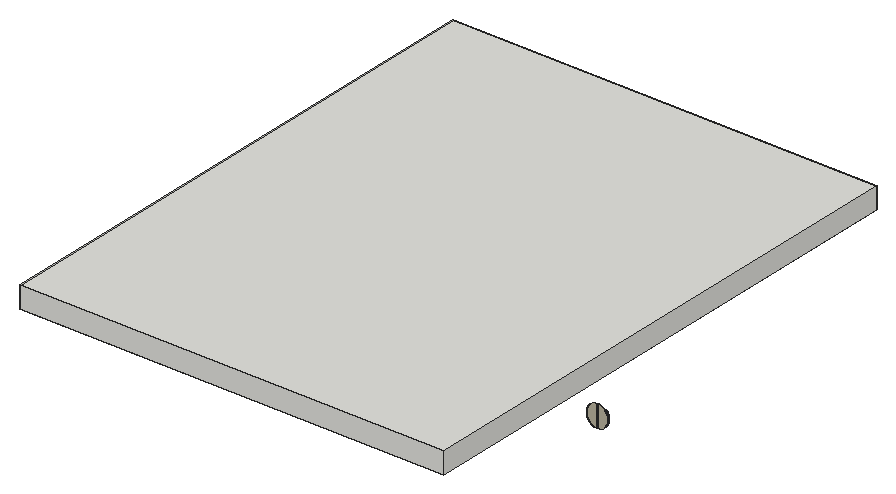
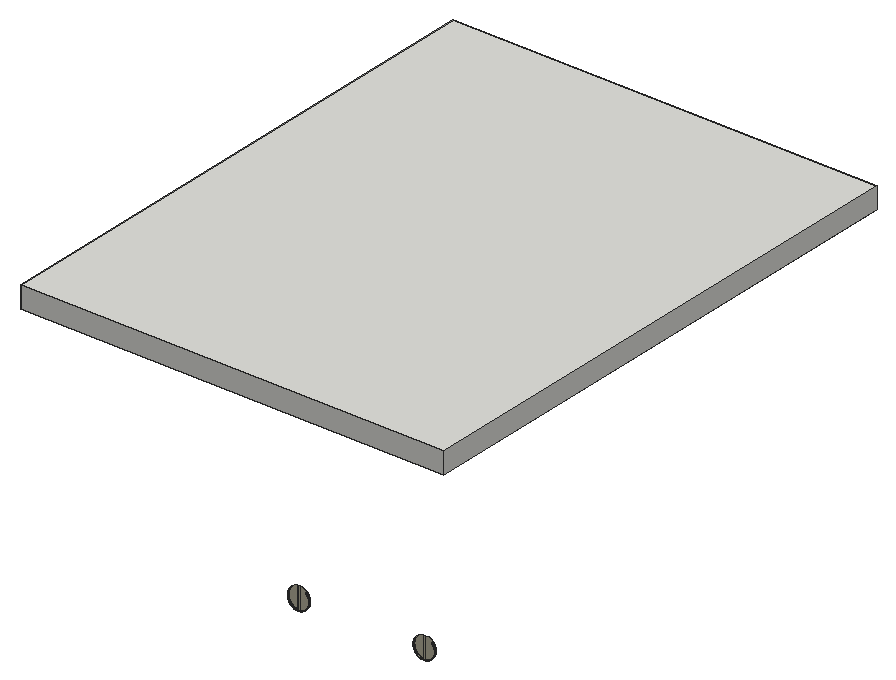
# SketchUp Ruby script. Lengths in millimetres.
U = 1.mm
M = Sketchup.active_model
def pt(a) = Geom::Point3d.new(a.map { |v| v * U })
def face(e, loops, mat)
  f = e.add_face(loops[0].map { |a| pt(a) })
  loops[1..].each { |l| e.add_face(l.map { |a| pt(a) }).erase! }
  f.material = f.back_material = mat if mat
  f
end
# faces: each face lists its corners as indices into pts; further lists are holes
def faces(e, pts, list, mat = nil) = list.each { |f| face(e, (f[0].is_a?(Array) ? f : [f]).map { |l| l.map { |i| pts[i] } }, mat) }
# xy, xz, yz: faces in a plane at the given z, y or x. An outline is a flat list of corners, or four numbers for a rectangle; further outlines are holes
def ring(l) = l.size == 4 ? [[l[0], l[1]], [l[2], l[1]], [l[2], l[3]], [l[0], l[3]]] : l.each_slice(2).to_a
def flat(e, list, mat, &to3) = list.each { |f| face(e, (f[0].is_a?(Array) ? f : [f]).map { |l| ring(l).map { |u, v| to3.(u, v) } }, mat) }
def xy(e, z, list, mat = nil) = flat(e, list, mat) { |x, y| [x, y, z] }
def xz(e, y, list, mat = nil) = flat(e, list, mat) { |x, z| [x, y, z] }
def yz(e, x, list, mat = nil) = flat(e, list, mat) { |y, z| [x, y, z] }
def lines(e, pts, list) = list.each { |a, b| e.add_line(pt(pts[a]), pt(pts[b])) }
# prism: a flat outline (further loops are holes) pulled along v
def prism(e, loops, v, mat = nil)
  f = face(e, loops, mat); d = Geom::Vector3d.new(v.map { |x| x * U })
  f.pushpull(f.normal.samedirection?(d) ? d.length : -d.length)
end
def box(e, o, s, mat = nil) = prism(e, [[o, [o[0] + s[0], o[1], o[2]], [o[0] + s[0], o[1] + s[1], o[2]], [o[0], o[1] + s[1], o[2]]]], [0, 0, s[2]], mat)
def at(x, y, z, deg = 0) = Geom::Transformation.translation(pt([x, y, z])) * Geom::Transformation.rotation(ORIGIN, Z_AXIS, deg.degrees)
def axes(o, x, y, z) = Geom::Transformation.new([*x, 0, *y, 0, *z, 0, *pt(o).to_a, 1])
def part(name) = M.definitions.add(name)
# library, detail: a bought-in or finely detailed component or shape, given as its bounding box
def library(name, o, s) = part(name).tap { |d| box(d.entities, o, s) }
def detail(e, o, s) = box(e.add_group.entities, o, s)
def put(e, d, t, mat = nil) = e.add_instance(d, t).tap { |i| i.material = mat if mat }
def group(e, t, mat = nil) = e.add_group.tap { |g| g.transformation = t; g.material = mat if mat }.entities
root = M.entities
M.materials.add("Uniboard-L19-Putty-4K").color = [187, 181, 160]
M.materials.add("[Color M09]").color = [0, 0, 0]
c1 = part("Group\#7")
detail(c1.entities,[0,0,0],[98.4,98.4,20])
xy(root,1219.2,[[604.4,3403.6,618.1,3413.6],[621.1,3403.6,634.7,3413.6],[1510.3,3403.6,1524,3413.6],[1527,3403.6,1540.7,3413.6]],"Uniboard-L19-Putty-4K")
xy(root,2871.6,[[1998,3403.6,2410.4,3412.6],[2449.4,3403.6,2861.9,3412.6]],"[Color M09]")
xz(root,3403.6,[[604.4,1219.2,618.1,1219.2,618.1,1371.6,604.4,1371.6,602.6,1371.2,600.2,1370.7,595.6,1369.3,593.2,1368.5,591,1367.6,588.7,1366.7,586.5,1365.7,582.1,1363.5,580,1362.3,577.9,1361,575.9,1359.7,573.9,1358.3,571.9,1356.8,570,1355.3,568.2,1353.7,564.6,1350.3,562.9,1348.6,561.3,1346.8,559.7,1344.9,556.7,1341.1,555.3,1339.1,554,1337,552.7,1335,551.5,1332.8,550.3,1330.7,548.3,1326.3,547.3,1324,545.7,1319.4,545,1317.1,544.3,1314.7,543.7,1312.3,543.2,1310,542.8,1307.6,542.5,1305.1,542.2,1302.7,542,1300.3,541.9,1297.8,541.9,1293,542,1290.5,542.2,1288.1,542.5,1285.7,542.8,1283.2,543.2,1280.8,543.7,1278.5,544.3,1276.1,545,1273.7,545.7,1271.4,547.3,1266.8,548.3,1264.5,550.3,1260.1,551.5,1258,552.7,1255.8,554,1253.8,555.3,1251.7,556.7,1249.7,559.7,1245.9,561.3,1244,562.9,1242.2,564.6,1240.5,568.2,1237.1,570,1235.5,571.9,1234,573.9,1232.5,575.9,1231.1,577.9,1229.8,580,1228.5,582.1,1227.3,586.5,1225.1,588.7,1224.1,591,1223.2,593.2,1222.3,595.6,1221.5,600.2,1220.1,602.6,1219.6],[621.1,1219.2,634.7,1219.2,636.5,1219.6,638.9,1220.1,641.2,1220.8,643.6,1221.5,645.9,1222.3,648.2,1223.2,650.4,1224.1,652.6,1225.1,657,1227.3,659.1,1228.5,661.2,1229.8,663.2,1231.1,665.2,1232.5,667.2,1234,669.1,1235.5,671,1237.1,672.8,1238.8,676.2,1242.2,677.9,1244,679.4,1245.9,681,1247.8,682.4,1249.7,683.8,1251.7,685.2,1253.8,686.4,1255.8,687.7,1258,688.8,1260.1,689.9,1262.3,690.9,1264.5,692.7,1269.1,693.5,1271.4,694.2,1273.7,695.4,1278.5,695.9,1280.8,696.3,1283.2,696.7,1285.7,697.1,1290.5,697.2,1293,697.3,1295.4,697.2,1297.8,697.1,1300.3,696.7,1305.1,696.3,1307.6,695.9,1310,695.4,1312.3,694.2,1317.1,693.5,1319.4,692.7,1321.7,690.9,1326.3,689.9,1328.5,688.8,1330.7,687.7,1332.8,686.4,1335,685.2,1337,683.8,1339.1,682.4,1341.1,681,1343,679.4,1344.9,677.9,1346.8,676.2,1348.6,672.8,1352,671,1353.7,669.1,1355.3,667.2,1356.8,665.2,1358.3,663.2,1359.7,661.2,1361,659.1,1362.3,657,1363.5,652.6,1365.7,650.4,1366.7,648.2,1367.6,645.9,1368.5,643.6,1369.3,641.2,1370,638.9,1370.7,636.5,1371.2,634.7,1371.6,621.1,1371.6],[1510.3,1219.2,1524,1219.2,1524,1371.6,1510.3,1371.6,1508.6,1371.2,1506.2,1370.7,1503.8,1370,1501.5,1369.3,1499.2,1368.5,1494.6,1366.7,1492.4,1365.7,1490.2,1364.6,1488.1,1363.5,1485.9,1362.3,1483.9,1361,1481.8,1359.7,1479.8,1358.3,1476,1355.3,1474.1,1353.7,1472.3,1352,1468.9,1348.6,1467.2,1346.8,1465.6,1344.9,1462.6,1341.1,1461.2,1339.1,1459.9,1337,1458.6,1335,1457.4,1332.8,1456.3,1330.7,1455.2,1328.5,1454.2,1326.3,1452.4,1321.7,1451.6,1319.4,1450.9,1317.1,1450.2,1314.7,1449.7,1312.3,1449.2,1310,1448.8,1307.6,1448.4,1305.1,1448.1,1302.7,1448,1300.3,1447.8,1297.8,1447.8,1293,1448,1290.5,1448.1,1288.1,1448.4,1285.7,1448.8,1283.2,1449.2,1280.8,1449.7,1278.5,1450.2,1276.1,1450.9,1273.7,1451.6,1271.4,1452.4,1269.1,1454.2,1264.5,1455.2,1262.3,1456.3,1260.1,1457.4,1258,1458.6,1255.8,1459.9,1253.8,1461.2,1251.7,1462.6,1249.7,1465.6,1245.9,1467.2,1244,1468.9,1242.2,1472.3,1238.8,1474.1,1237.1,1476,1235.5,1479.8,1232.5,1481.8,1231.1,1483.9,1229.8,1485.9,1228.5,1488.1,1227.3,1490.2,1226.2,1492.4,1225.1,1494.6,1224.1,1499.2,1222.3,1501.5,1221.5,1503.8,1220.8,1506.2,1220.1,1508.6,1219.6],[1527,1219.2,1540.7,1219.2,1542.4,1219.6,1544.8,1220.1,1547.2,1220.8,1549.5,1221.5,1551.8,1222.3,1556.4,1224.1,1558.6,1225.1,1560.8,1226.2,1562.9,1227.3,1565.1,1228.5,1567.1,1229.8,1569.2,1231.1,1571.2,1232.5,1575,1235.5,1576.9,1237.1,1578.7,1238.8,1582.1,1242.2,1583.8,1244,1585.4,1245.9,1588.4,1249.7,1589.8,1251.7,1591.1,1253.8,1592.4,1255.8,1593.6,1258,1594.7,1260.1,1595.8,1262.3,1596.8,1264.5,1598.6,1269.1,1599.4,1271.4,1600.1,1273.7,1600.8,1276.1,1601.3,1278.5,1601.8,1280.8,1602.2,1283.2,1602.6,1285.7,1602.9,1288.1,1603,1290.5,1603.2,1293,1603.2,1297.8,1603,1300.3,1602.9,1302.7,1602.6,1305.1,1602.2,1307.6,1601.8,1310,1601.3,1312.3,1600.8,1314.7,1600.1,1317.1,1599.4,1319.4,1598.6,1321.7,1596.8,1326.3,1595.8,1328.5,1594.7,1330.7,1593.6,1332.8,1592.4,1335,1591.1,1337,1589.8,1339.1,1588.4,1341.1,1585.4,1344.9,1583.8,1346.8,1582.1,1348.6,1578.7,1352,1576.9,1353.7,1575,1355.3,1571.2,1358.3,1569.2,1359.7,1567.1,1361,1565.1,1362.3,1562.9,1363.5,1560.8,1364.6,1558.6,1365.7,1556.4,1366.7,1551.8,1368.5,1549.5,1369.3,1547.2,1370,1544.8,1370.7,1542.4,1371.2,1540.7,1371.6,1527,1371.6]],"Uniboard-L19-Putty-4K")
yz(root,541.9,[[3403.6,1293,3413.6,1295.4],[3403.6,1295.4,3413.6,1297.8]],"Uniboard-L19-Putty-4K")
yz(root,618.1,[[3403.6,1219.2,3413.6,1371.6]],"Uniboard-L19-Putty-4K")
yz(root,621.1,[[3403.6,1219.2,3413.6,1371.6]],"Uniboard-L19-Putty-4K")
yz(root,1447.8,[[3403.6,1293,3413.6,1295.4],[3403.6,1295.4,3413.6,1297.8]],"Uniboard-L19-Putty-4K")
yz(root,1524,[[3403.6,1219.2,3413.6,1371.6]],"Uniboard-L19-Putty-4K")
yz(root,1527,[[3403.6,1219.2,3413.6,1371.6]],"Uniboard-L19-Putty-4K")
yz(root,1603.2,[[3403.6,1293,3413.6,1295.4],[3403.6,1295.4,3413.6,1297.8]])
p = [[602.6,3413.6,1219.6],[604.4,3413.6,1219.2],[604.4,3403.6,1219.2],[602.6,3403.6,1219.6],[634.7,3413.6,1219.2],[636.5,3413.6,1219.6],
  [636.5,3403.6,1219.6],[634.7,3403.6,1219.2],[1508.6,3413.6,1219.6],[1510.3,3413.6,1219.2],[1510.3,3403.6,1219.2],[1508.6,3403.6,1219.6],
  [1540.7,3413.6,1219.2],[1542.4,3413.6,1219.6],[1542.4,3403.6,1219.6],[1540.7,3403.6,1219.2],[600.2,3413.6,1220.1],[600.2,3403.6,1220.1],
  [638.9,3413.6,1220.1],[638.9,3403.6,1220.1],[1506.2,3413.6,1220.1],[1506.2,3403.6,1220.1],[1544.8,3413.6,1220.1],[1544.8,3403.6,1220.1],
  [597.9,3413.6,1220.8],[597.9,3403.6,1220.8],[641.2,3413.6,1220.8],[641.2,3403.6,1220.8],[1503.8,3413.6,1220.8],[1503.8,3403.6,1220.8],
  [1547.2,3413.6,1220.8],[1547.2,3403.6,1220.8],[595.6,3413.6,1221.5],[595.6,3403.6,1221.5],[643.6,3413.6,1221.5],[643.6,3403.6,1221.5],
  [1501.5,3413.6,1221.5],[1501.5,3403.6,1221.5],[1549.5,3413.6,1221.5],[1549.5,3403.6,1221.5],[593.2,3413.6,1222.3],[593.2,3403.6,1222.3],
  [645.9,3413.6,1222.3],[645.9,3403.6,1222.3],[1499.2,3413.6,1222.3],[1499.2,3403.6,1222.3],[1551.8,3413.6,1222.3],[1551.8,3403.6,1222.3],
  [591,3413.6,1223.2],[591,3403.6,1223.2],[648.2,3413.6,1223.2],[648.2,3403.6,1223.2],[1496.9,3413.6,1223.2],[1496.9,3403.6,1223.2],
  [1554.1,3413.6,1223.2],[1554.1,3403.6,1223.2],[588.7,3413.6,1224.1],[588.7,3403.6,1224.1],[650.4,3413.6,1224.1],[650.4,3403.6,1224.1],
  [1494.6,3413.6,1224.1],[1494.6,3403.6,1224.1],[1556.4,3413.6,1224.1],[1556.4,3403.6,1224.1],[586.5,3413.6,1225.1],[586.5,3403.6,1225.1],
  [652.6,3413.6,1225.1],[652.6,3403.6,1225.1],[1492.4,3413.6,1225.1],[1492.4,3403.6,1225.1],[1558.6,3413.6,1225.1],[1558.6,3403.6,1225.1],
  [584.3,3413.6,1226.2],[584.3,3403.6,1226.2],[654.8,3413.6,1226.2],[654.8,3403.6,1226.2],[1490.2,3413.6,1226.2],[1490.2,3403.6,1226.2],
  [1560.8,3413.6,1226.2],[1560.8,3403.6,1226.2],[582.1,3413.6,1227.3],[582.1,3403.6,1227.3],[657,3413.6,1227.3],[657,3403.6,1227.3],
  [1488.1,3413.6,1227.3],[1488.1,3403.6,1227.3],[1562.9,3413.6,1227.3],[1562.9,3403.6,1227.3],[580,3413.6,1228.5],[580,3403.6,1228.5],
  [659.1,3413.6,1228.5],[659.1,3403.6,1228.5],[1485.9,3413.6,1228.5],[1485.9,3403.6,1228.5],[1565.1,3413.6,1228.5],[1565.1,3403.6,1228.5],
  [577.9,3413.6,1229.8],[577.9,3403.6,1229.8],[661.2,3413.6,1229.8],[661.2,3403.6,1229.8],[1483.9,3413.6,1229.8],[1483.9,3403.6,1229.8],
  [1567.1,3413.6,1229.8],[1567.1,3403.6,1229.8],[575.9,3413.6,1231.1],[575.9,3403.6,1231.1],[663.2,3413.6,1231.1],[663.2,3403.6,1231.1],
  [1481.8,3413.6,1231.1],[1481.8,3403.6,1231.1],[1569.2,3413.6,1231.1],[1569.2,3403.6,1231.1],[573.9,3413.6,1232.5],[573.9,3403.6,1232.5],
  [665.2,3413.6,1232.5],[665.2,3403.6,1232.5],[1479.8,3413.6,1232.5],[1479.8,3403.6,1232.5],[1571.2,3413.6,1232.5],[1571.2,3403.6,1232.5],
  [571.9,3413.6,1234],[571.9,3403.6,1234],[667.2,3413.6,1234],[667.2,3403.6,1234],[1477.9,3413.6,1234],[1477.9,3403.6,1234],
  [1573.1,3413.6,1234],[1573.1,3403.6,1234],[570,3413.6,1235.5],[570,3403.6,1235.5],[669.1,3413.6,1235.5],[669.1,3403.6,1235.5],
  [1476,3413.6,1235.5],[1476,3403.6,1235.5],[1575,3413.6,1235.5],[1575,3403.6,1235.5],[568.2,3413.6,1237.1],[568.2,3403.6,1237.1],
  [671,3413.6,1237.1],[671,3403.6,1237.1],[1474.1,3413.6,1237.1],[1474.1,3403.6,1237.1],[1576.9,3413.6,1237.1],[1576.9,3403.6,1237.1],
  [566.4,3413.6,1238.8],[566.4,3403.6,1238.8],[672.8,3413.6,1238.8],[672.8,3403.6,1238.8],[1472.3,3413.6,1238.8],[1472.3,3403.6,1238.8],
  [1578.7,3413.6,1238.8],[1578.7,3403.6,1238.8],[564.6,3413.6,1240.5],[564.6,3403.6,1240.5],[674.5,3413.6,1240.5],[674.5,3403.6,1240.5],
  [1470.6,3413.6,1240.5],[1470.6,3403.6,1240.5],[1580.4,3413.6,1240.5],[1580.4,3403.6,1240.5],[562.9,3413.6,1242.2],[562.9,3403.6,1242.2],
  [676.2,3413.6,1242.2],[676.2,3403.6,1242.2],[1468.9,3413.6,1242.2],[1468.9,3403.6,1242.2],[1582.1,3413.6,1242.2],[1582.1,3403.6,1242.2],
  [561.3,3413.6,1244],[561.3,3403.6,1244],[677.9,3413.6,1244],[677.9,3403.6,1244],[1467.2,3413.6,1244],[1467.2,3403.6,1244],
  [1583.8,3413.6,1244],[1583.8,3403.6,1244],[559.7,3413.6,1245.9],[559.7,3403.6,1245.9],[679.4,3413.6,1245.9],[679.4,3403.6,1245.9],
  [1465.6,3413.6,1245.9],[1465.6,3403.6,1245.9],[1585.4,3413.6,1245.9],[1585.4,3403.6,1245.9],[558.2,3413.6,1247.8],[558.2,3403.6,1247.8],
  [681,3413.6,1247.8],[681,3403.6,1247.8],[1464.1,3413.6,1247.8],[1464.1,3403.6,1247.8],[1586.9,3413.6,1247.8],[1586.9,3403.6,1247.8],
  [556.7,3413.6,1249.7],[556.7,3403.6,1249.7],[682.4,3413.6,1249.7],[682.4,3403.6,1249.7],[1462.6,3413.6,1249.7],[1462.6,3403.6,1249.7],
  [1588.4,3413.6,1249.7],[1588.4,3403.6,1249.7],[555.3,3413.6,1251.7],[555.3,3403.6,1251.7],[683.8,3413.6,1251.7],[683.8,3403.6,1251.7],
  [1461.2,3413.6,1251.7],[1461.2,3403.6,1251.7],[1589.8,3413.6,1251.7],[1589.8,3403.6,1251.7],[554,3413.6,1253.8],[554,3403.6,1253.8],
  [685.2,3413.6,1253.8],[685.2,3403.6,1253.8],[1459.9,3413.6,1253.8],[1459.9,3403.6,1253.8],[1591.1,3413.6,1253.8],[1591.1,3403.6,1253.8],
  [552.7,3413.6,1255.8],[552.7,3403.6,1255.8],[686.4,3413.6,1255.8],[686.4,3403.6,1255.8],[1458.6,3413.6,1255.8],[1458.6,3403.6,1255.8],
  [1592.4,3413.6,1255.8],[1592.4,3403.6,1255.8],[551.5,3413.6,1258],[551.5,3403.6,1258],[687.7,3413.6,1258],[687.7,3403.6,1258],
  [1457.4,3413.6,1258],[1457.4,3403.6,1258],[1593.6,3413.6,1258],[1593.6,3403.6,1258],[550.3,3413.6,1260.1],[550.3,3403.6,1260.1],
  [688.8,3413.6,1260.1],[688.8,3403.6,1260.1],[1456.3,3413.6,1260.1],[1456.3,3403.6,1260.1],[1594.7,3413.6,1260.1],[1594.7,3403.6,1260.1],
  [549.3,3413.6,1262.3],[549.3,3403.6,1262.3],[689.9,3413.6,1262.3],[689.9,3403.6,1262.3],[1455.2,3413.6,1262.3],[1455.2,3403.6,1262.3],
  [1595.8,3413.6,1262.3],[1595.8,3403.6,1262.3],[548.3,3413.6,1264.5],[548.3,3403.6,1264.5],[690.9,3413.6,1264.5],[690.9,3403.6,1264.5],
  [1454.2,3413.6,1264.5],[1454.2,3403.6,1264.5],[1596.8,3413.6,1264.5],[1596.8,3403.6,1264.5],[547.3,3413.6,1266.8],[547.3,3403.6,1266.8],
  [691.8,3413.6,1266.8],[691.8,3403.6,1266.8],[1453.3,3413.6,1266.8],[1453.3,3403.6,1266.8],[1597.7,3413.6,1266.8],[1597.7,3403.6,1266.8],
  [546.5,3413.6,1269.1],[546.5,3403.6,1269.1],[692.7,3413.6,1269.1],[692.7,3403.6,1269.1],[1452.4,3413.6,1269.1],[1452.4,3403.6,1269.1],
  [1598.6,3413.6,1269.1],[1598.6,3403.6,1269.1],[545.7,3413.6,1271.4],[545.7,3403.6,1271.4],[693.5,3413.6,1271.4],[693.5,3403.6,1271.4],
  [1451.6,3413.6,1271.4],[1451.6,3403.6,1271.4],[1599.4,3413.6,1271.4],[1599.4,3403.6,1271.4],[545,3413.6,1273.7],[545,3403.6,1273.7],
  [694.2,3413.6,1273.7],[694.2,3403.6,1273.7],[1450.9,3413.6,1273.7],[1450.9,3403.6,1273.7],[1600.1,3413.6,1273.7],[1600.1,3403.6,1273.7],
  [544.3,3413.6,1276.1],[544.3,3403.6,1276.1],[694.8,3413.6,1276.1],[694.8,3403.6,1276.1],[1450.2,3413.6,1276.1],[1450.2,3403.6,1276.1],
  [1600.8,3413.6,1276.1],[1600.8,3403.6,1276.1],[543.7,3413.6,1278.5],[543.7,3403.6,1278.5],[695.4,3413.6,1278.5],[695.4,3403.6,1278.5],
  [1449.7,3413.6,1278.5],[1449.7,3403.6,1278.5],[1601.3,3413.6,1278.5],[1601.3,3403.6,1278.5],[543.2,3413.6,1280.8],[543.2,3403.6,1280.8],
  [695.9,3413.6,1280.8],[695.9,3403.6,1280.8],[1449.2,3413.6,1280.8],[1449.2,3403.6,1280.8],[1601.8,3413.6,1280.8],[1601.8,3403.6,1280.8],
  [542.8,3413.6,1283.2],[542.8,3403.6,1283.2],[696.3,3413.6,1283.2],[696.3,3403.6,1283.2],[1448.8,3413.6,1283.2],[1448.8,3403.6,1283.2],
  [1602.2,3413.6,1283.2],[1602.2,3403.6,1283.2],[542.5,3413.6,1285.7],[542.5,3403.6,1285.7],[696.7,3413.6,1285.7],[696.7,3403.6,1285.7],
  [1448.4,3413.6,1285.7],[1448.4,3403.6,1285.7],[1602.6,3413.6,1285.7],[1602.6,3403.6,1285.7],[542.2,3413.6,1288.1],[542.2,3403.6,1288.1],
  [696.9,3413.6,1288.1],[696.9,3403.6,1288.1],[1448.1,3413.6,1288.1],[1448.1,3403.6,1288.1],[1602.9,3413.6,1288.1],[1602.9,3403.6,1288.1],
  [542,3413.6,1290.5],[542,3403.6,1290.5],[697.1,3413.6,1290.5],[697.1,3403.6,1290.5],[1448,3413.6,1290.5],[1448,3403.6,1290.5],
  [1603,3413.6,1290.5],[1603,3403.6,1290.5],[541.9,3413.6,1293],[541.9,3403.6,1293],[697.2,3413.6,1293],[697.2,3403.6,1293],
  [1447.8,3413.6,1293],[1447.8,3403.6,1293],[1603.2,3413.6,1293],[1603.2,3403.6,1293],[697.3,3413.6,1295.4],[697.3,3403.6,1295.4],
  [697.2,3413.6,1297.8],[697.2,3403.6,1297.8],[542,3413.6,1300.3],[541.9,3413.6,1297.8],[541.9,3403.6,1297.8],[542,3403.6,1300.3],
  [697.1,3413.6,1300.3],[697.1,3403.6,1300.3],[1448,3413.6,1300.3],[1447.8,3413.6,1297.8],[1447.8,3403.6,1297.8],[1448,3403.6,1300.3],
  [1603.2,3413.6,1297.8],[1603,3413.6,1300.3],[1603,3403.6,1300.3],[1603.2,3403.6,1297.8],[542.2,3413.6,1302.7],[542.2,3403.6,1302.7],
  [696.9,3413.6,1302.7],[696.9,3403.6,1302.7],[1448.1,3413.6,1302.7],[1448.1,3403.6,1302.7],[1602.9,3413.6,1302.7],[1602.9,3403.6,1302.7],
  [542.5,3413.6,1305.1],[542.5,3403.6,1305.1],[696.7,3413.6,1305.1],[696.7,3403.6,1305.1],[1448.4,3413.6,1305.1],[1448.4,3403.6,1305.1],
  [1602.6,3413.6,1305.1],[1602.6,3403.6,1305.1],[542.8,3413.6,1307.6],[542.8,3403.6,1307.6],[696.3,3413.6,1307.6],[696.3,3403.6,1307.6],
  [1448.8,3413.6,1307.6],[1448.8,3403.6,1307.6],[1602.2,3413.6,1307.6],[1602.2,3403.6,1307.6],[543.2,3413.6,1310],[543.2,3403.6,1310],
  [695.9,3413.6,1310],[695.9,3403.6,1310],[1449.2,3413.6,1310],[1449.2,3403.6,1310],[1601.8,3413.6,1310],[1601.8,3403.6,1310],
  [543.7,3413.6,1312.3],[543.7,3403.6,1312.3],[695.4,3413.6,1312.3],[695.4,3403.6,1312.3],[1449.7,3413.6,1312.3],[1449.7,3403.6,1312.3],
  [1601.3,3413.6,1312.3],[1601.3,3403.6,1312.3],[544.3,3413.6,1314.7],[544.3,3403.6,1314.7],[694.8,3413.6,1314.7],[694.8,3403.6,1314.7],
  [1450.2,3413.6,1314.7],[1450.2,3403.6,1314.7],[1600.8,3413.6,1314.7],[1600.8,3403.6,1314.7],[545,3413.6,1317.1],[545,3403.6,1317.1],
  [694.2,3413.6,1317.1],[694.2,3403.6,1317.1],[1450.9,3413.6,1317.1],[1450.9,3403.6,1317.1],[1600.1,3413.6,1317.1],[1600.1,3403.6,1317.1],
  [545.7,3413.6,1319.4],[545.7,3403.6,1319.4],[693.5,3413.6,1319.4],[693.5,3403.6,1319.4],[1451.6,3413.6,1319.4],[1451.6,3403.6,1319.4],
  [1599.4,3413.6,1319.4],[1599.4,3403.6,1319.4],[546.5,3413.6,1321.7],[546.5,3403.6,1321.7],[692.7,3413.6,1321.7],[692.7,3403.6,1321.7],
  [1452.4,3413.6,1321.7],[1452.4,3403.6,1321.7],[1598.6,3413.6,1321.7],[1598.6,3403.6,1321.7],[547.3,3413.6,1324],[547.3,3403.6,1324],
  [691.8,3413.6,1324],[691.8,3403.6,1324],[1453.3,3413.6,1324],[1453.3,3403.6,1324],[1597.7,3413.6,1324],[1597.7,3403.6,1324],
  [548.3,3413.6,1326.3],[548.3,3403.6,1326.3],[690.9,3413.6,1326.3],[690.9,3403.6,1326.3],[1454.2,3413.6,1326.3],[1454.2,3403.6,1326.3],
  [1596.8,3413.6,1326.3],[1596.8,3403.6,1326.3],[549.3,3413.6,1328.5],[549.3,3403.6,1328.5],[689.9,3413.6,1328.5],[689.9,3403.6,1328.5],
  [1455.2,3413.6,1328.5],[1455.2,3403.6,1328.5],[1595.8,3413.6,1328.5],[1595.8,3403.6,1328.5],[550.3,3413.6,1330.7],[550.3,3403.6,1330.7],
  [688.8,3413.6,1330.7],[688.8,3403.6,1330.7],[1456.3,3413.6,1330.7],[1456.3,3403.6,1330.7],[1594.7,3413.6,1330.7],[1594.7,3403.6,1330.7],
  [551.5,3413.6,1332.8],[551.5,3403.6,1332.8],[687.7,3413.6,1332.8],[687.7,3403.6,1332.8],[1457.4,3413.6,1332.8],[1457.4,3403.6,1332.8],
  [1593.6,3413.6,1332.8],[1593.6,3403.6,1332.8],[552.7,3413.6,1335],[552.7,3403.6,1335],[686.4,3413.6,1335],[686.4,3403.6,1335],
  [1458.6,3413.6,1335],[1458.6,3403.6,1335],[1592.4,3413.6,1335],[1592.4,3403.6,1335],[554,3413.6,1337],[554,3403.6,1337],
  [685.2,3413.6,1337],[685.2,3403.6,1337],[1459.9,3413.6,1337],[1459.9,3403.6,1337],[1591.1,3413.6,1337],[1591.1,3403.6,1337],
  [555.3,3413.6,1339.1],[555.3,3403.6,1339.1],[683.8,3413.6,1339.1],[683.8,3403.6,1339.1],[1461.2,3413.6,1339.1],[1461.2,3403.6,1339.1],
  [1589.8,3413.6,1339.1],[1589.8,3403.6,1339.1],[556.7,3413.6,1341.1],[556.7,3403.6,1341.1],[682.4,3413.6,1341.1],[682.4,3403.6,1341.1],
  [1462.6,3413.6,1341.1],[1462.6,3403.6,1341.1],[1588.4,3413.6,1341.1],[1588.4,3403.6,1341.1],[558.2,3413.6,1343],[558.2,3403.6,1343],
  [681,3413.6,1343],[681,3403.6,1343],[1464.1,3413.6,1343],[1464.1,3403.6,1343],[1586.9,3413.6,1343],[1586.9,3403.6,1343],
  [559.7,3413.6,1344.9],[559.7,3403.6,1344.9],[679.4,3413.6,1344.9],[679.4,3403.6,1344.9],[1465.6,3413.6,1344.9],[1465.6,3403.6,1344.9],
  [1585.4,3413.6,1344.9],[1585.4,3403.6,1344.9],[561.3,3413.6,1346.8],[561.3,3403.6,1346.8],[677.9,3413.6,1346.8],[677.9,3403.6,1346.8],
  [1467.2,3413.6,1346.8],[1467.2,3403.6,1346.8],[1583.8,3413.6,1346.8],[1583.8,3403.6,1346.8],[562.9,3413.6,1348.6],[562.9,3403.6,1348.6],
  [676.2,3413.6,1348.6],[676.2,3403.6,1348.6],[1468.9,3413.6,1348.6],[1468.9,3403.6,1348.6],[1582.1,3413.6,1348.6],[1582.1,3403.6,1348.6],
  [564.6,3413.6,1350.3],[564.6,3403.6,1350.3],[674.5,3413.6,1350.3],[674.5,3403.6,1350.3],[1470.6,3413.6,1350.3],[1470.6,3403.6,1350.3],
  [1580.4,3413.6,1350.3],[1580.4,3403.6,1350.3],[1472.3,3413.6,1352],[1472.3,3403.6,1352],[1578.7,3413.6,1352],[1578.7,3403.6,1352],
  [1524,3403.6,1752.6],[1527,3403.6,1752.6]]
faces(root,p,[[0,1,2,3],[4,5,6,7],[8,9,10,11],[16,0,3,17],[5,18,19,6],[20,8,11,21],[24,16,17,25],[18,26,27,19],
  [28,20,21,29],[32,24,25,33],[26,34,35,27],[36,28,29,37],[40,32,33,41],[34,42,43,35],[44,36,37,45],[48,40,41,49],
  [42,50,51,43],[52,44,45,53],[56,48,49,57],[50,58,59,51],[60,52,53,61],[64,56,57,65],[58,66,67,59],[68,60,61,69],
  [72,64,65,73],[66,74,75,67],[76,68,69,77],[80,72,73,81],[74,82,83,75],[84,76,77,85],[88,80,81,89],[82,90,91,83],
  [92,84,85,93],[96,88,89,97],[90,98,99,91],[100,92,93,101],[104,96,97,105],[98,106,107,99],[108,100,101,109],[112,104,105,113],
  [106,114,115,107],[116,108,109,117],[120,112,113,121],[114,122,123,115],[124,116,117,125],[128,120,121,129],[122,130,131,123],[132,124,125,133],
  [136,128,129,137],[130,138,139,131],[140,132,133,141],[144,136,137,145],[138,146,147,139],[148,140,141,149],[152,144,145,153],[146,154,155,147],
  [156,148,149,157],[160,152,153,161],[154,162,163,155],[164,156,157,165],[168,160,161,169],[162,170,171,163],[172,164,165,173],[176,168,169,177],
  [170,178,179,171],[180,172,173,181],[184,176,177,185],[178,186,187,179],[188,180,181,189],[192,184,185,193],[186,194,195,187],[196,188,189,197],
  [200,192,193,201],[194,202,203,195],[204,196,197,205],[208,200,201,209],[202,210,211,203],[212,204,205,213],[216,208,209,217],[210,218,219,211],
  [220,212,213,221],[224,216,217,225],[218,226,227,219],[228,220,221,229],[232,224,225,233],[226,234,235,227],[236,228,229,237],[240,232,233,241],
  [234,242,243,235],[244,236,237,245],[248,240,241,249],[242,250,251,243],[252,244,245,253],[256,248,249,257],[250,258,259,251],[260,252,253,261],
  [264,256,257,265],[258,266,267,259],[268,260,261,269],[272,264,265,273],[266,274,275,267],[276,268,269,277],[280,272,273,281],[274,282,283,275],
  [284,276,277,285],[288,280,281,289],[282,290,291,283],[292,284,285,293],[296,288,289,297],[290,298,299,291],[300,292,293,301],[304,296,297,305],
  [298,306,307,299],[308,300,301,309],[312,304,305,313],[306,314,315,307],[316,308,309,317],[320,312,313,321],[314,322,323,315],[324,316,317,325],
  [328,320,321,329],[322,330,331,323],[332,324,325,333],[336,328,329,337],[330,338,339,331],[340,332,333,341],[344,336,337,345],[338,346,347,339],
  [348,340,341,349],[346,352,353,347],[352,354,355,353],[356,357,358,359],[354,360,361,355],[362,363,364,365],[370,356,359,371],[360,372,373,361],
  [374,362,365,375],[378,370,371,379],[372,380,381,373],[382,374,375,383],[386,378,379,387],[380,388,389,381],[390,382,383,391],[394,386,387,395],
  [388,396,397,389],[398,390,391,399],[402,394,395,403],[396,404,405,397],[406,398,399,407],[410,402,403,411],[404,412,413,405],[414,406,407,415],
  [418,410,411,419],[412,420,421,413],[422,414,415,423],[426,418,419,427],[420,428,429,421],[430,422,423,431],[434,426,427,435],[428,436,437,429],
  [438,430,431,439],[442,434,435,443],[436,444,445,437],[446,438,439,447],[450,442,443,451],[444,452,453,445],[454,446,447,455],[458,450,451,459],
  [452,460,461,453],[462,454,455,463],[466,458,459,467],[460,468,469,461],[470,462,463,471],[474,466,467,475],[468,476,477,469],[478,470,471,479],
  [482,474,475,483],[476,484,485,477],[486,478,479,487],[490,482,483,491],[484,492,493,485],[494,486,487,495],[498,490,491,499],[492,500,501,493],
  [502,494,495,503],[506,498,499,507],[500,508,509,501],[510,502,503,511],[514,506,507,515],[508,516,517,509],[518,510,511,519],[522,514,515,523],
  [516,524,525,517],[526,518,519,527],[530,522,523,531],[524,532,533,525],[534,526,527,535],[538,530,531,539],[532,540,541,533],[542,534,535,543],
  [546,538,539,547],[540,548,549,541],[550,542,543,551],[554,550,551,555]],"Uniboard-L19-Putty-4K")
faces(root,p,[[12,13,14,15],[13,22,23,14],[22,30,31,23],[30,38,39,31],[38,46,47,39],[46,54,55,47],[54,62,63,55],[62,70,71,63],
  [70,78,79,71],[78,86,87,79],[86,94,95,87],[94,102,103,95],[102,110,111,103],[110,118,119,111],[118,126,127,119],[126,134,135,127],
  [134,142,143,135],[142,150,151,143],[150,158,159,151],[158,166,167,159],[166,174,175,167],[174,182,183,175],[182,190,191,183],[190,198,199,191],
  [198,206,207,199],[206,214,215,207],[214,222,223,215],[222,230,231,223],[230,238,239,231],[238,246,247,239],[246,254,255,247],[254,262,263,255],
  [262,270,271,263],[270,278,279,271],[278,286,287,279],[286,294,295,287],[294,302,303,295],[302,310,311,303],[310,318,319,311],[318,326,327,319],
  [326,334,335,327],[334,342,343,335],[342,350,351,343],[366,367,368,369],[367,376,377,368],[376,384,385,377],[384,392,393,385],[392,400,401,393],
  [400,408,409,401],[408,416,417,409],[416,424,425,417],[424,432,433,425],[432,440,441,433],[440,448,449,441],[448,456,457,449],[456,464,465,457],
  [464,472,473,465],[472,480,481,473],[480,488,489,481],[488,496,497,489],[496,504,505,497],[504,512,513,505],[512,520,521,513],[520,528,529,521],
  [528,536,537,529],[536,544,545,537],[544,552,553,545],[552,556,557,553]])
lines(root,p,[[558,559]])
put(root,c1,at(2522.2,357.2,2875.6))
put(root,c1,at(1495.1,357.2,2875.6))
put(root,c1,at(564.9,357.2,2875.6))
put(root,c1,at(2522.2,916,2875.6))
put(root,c1,at(564.9,916,2875.6))
put(root,c1,at(2522.2,1525.6,2875.6))
put(root,c1,at(564.9,1525.6,2875.6))
g1 = group(root,at(0,965.2,2895.6))
xy(g1,0,[[[0,-850.9,3048,3048],[741.2,-420.1,2265.2,1697.6]],[766.6,-394.7,2239.8,1672.2]])
xy(g1,152.4,[[0,-850.9,3048,3048]])
xz(g1,-850.9,[[0,0,3048,152.4]])
xz(g1,3048,[[0,0,3048,152.4]])
yz(g1,0,[[-850.9,0,3048,152.4]])
yz(g1,3048,[[-850.9,0,3048,152.4]])
g2 = group(g1,at(741.2,-420.1,0))
xy(g2,0,[[[0,0,1524,2117.7],[25.4,25.4,1498.6,2092.3]]])
put(root,c1,at(2522.2,2135.2,2875.6))
put(root,c1,at(564.9,2135.2,2875.6))
g3 = group(root,at(582.2,2762.1,2885.6))
xy(g3,0,[[31.9,0,23.6,1.1,15.9,4.3,9.3,9.3,4.3,15.9,1.1,23.6,0,31.9,1.1,40.1,4.3,47.8,9.3,54.4,15.9,59.5,23.6,62.7,31.9,63.8,40.1,62.7,47.8,59.5,54.4,54.4,59.5,47.8,62.7,40.1,63.8,31.9,62.7,23.6,59.5,15.9,54.4,9.3,47.8,4.3,40.1,1.1]])
put(root,c1,at(564.9,2744.8,2875.6))
put(root,c1,at(1495.1,2744.8,2875.6))
put(root,c1,at(2522.2,2744.8,2875.6))
